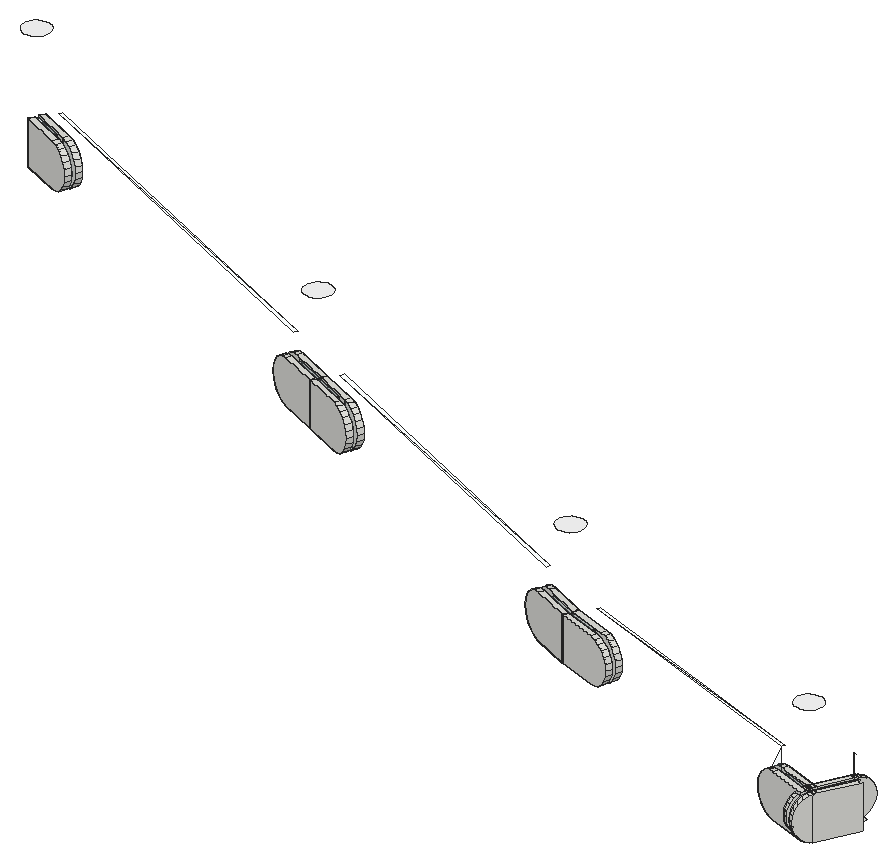
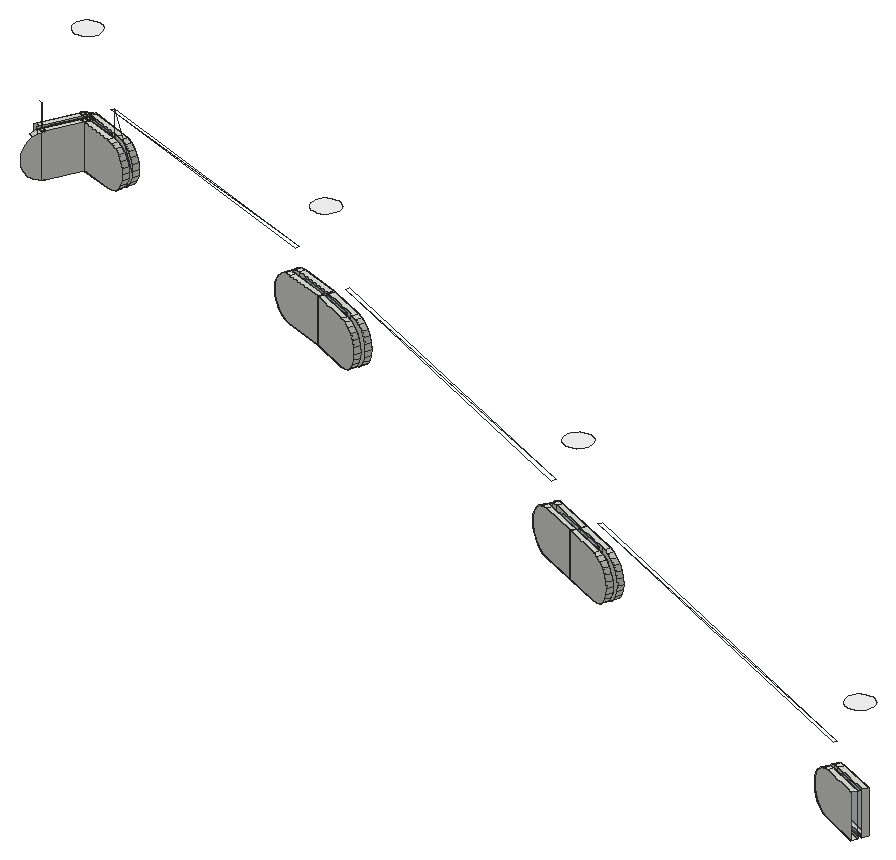
# SketchUp Ruby script. Lengths in inches.
U = 1.inch
M = Sketchup.active_model
def pt(a) = Geom::Point3d.new(a.map { |v| v * U })
def face(e, loops, mat)
  f = e.add_face(loops[0].map { |a| pt(a) })
  loops[1..].each { |l| e.add_face(l.map { |a| pt(a) }).erase! }
  f.material = f.back_material = mat if mat
  f
end
# faces: each face lists its corners as indices into pts; further lists are holes
def faces(e, pts, list, mat = nil) = list.each { |f| face(e, (f[0].is_a?(Array) ? f : [f]).map { |l| l.map { |i| pts[i] } }, mat) }
# xy, xz, yz: faces in a plane at the given z, y or x. An outline is a flat list of corners, or four numbers for a rectangle; further outlines are holes
def ring(l) = l.size == 4 ? [[l[0], l[1]], [l[2], l[1]], [l[2], l[3]], [l[0], l[3]]] : l.each_slice(2).to_a
def flat(e, list, mat, &to3) = list.each { |f| face(e, (f[0].is_a?(Array) ? f : [f]).map { |l| ring(l).map { |u, v| to3.(u, v) } }, mat) }
def xy(e, z, list, mat = nil) = flat(e, list, mat) { |x, y| [x, y, z] }
def xz(e, y, list, mat = nil) = flat(e, list, mat) { |x, z| [x, y, z] }
def yz(e, x, list, mat = nil) = flat(e, list, mat) { |y, z| [x, y, z] }
def lines(e, pts, list) = list.each { |a, b| e.add_line(pt(pts[a]), pt(pts[b])) }
# prism: a flat outline (further loops are holes) pulled along v
def prism(e, loops, v, mat = nil)
  f = face(e, loops, mat); d = Geom::Vector3d.new(v.map { |x| x * U })
  f.pushpull(f.normal.samedirection?(d) ? d.length : -d.length)
end
def box(e, o, s, mat = nil) = prism(e, [[o, [o[0] + s[0], o[1], o[2]], [o[0] + s[0], o[1] + s[1], o[2]], [o[0], o[1] + s[1], o[2]]]], [0, 0, s[2]], mat)
def at(x, y, z, deg = 0) = Geom::Transformation.translation(pt([x, y, z])) * Geom::Transformation.rotation(ORIGIN, Z_AXIS, deg.degrees)
def axes(o, x, y, z) = Geom::Transformation.new([*x, 0, *y, 0, *z, 0, *pt(o).to_a, 1])
def part(name) = M.definitions.add(name)
# library, detail: a bought-in or finely detailed component or shape, given as its bounding box
def library(name, o, s) = part(name).tap { |d| box(d.entities, o, s) }
def detail(e, o, s) = box(e.add_group.entities, o, s)
def put(e, d, t, mat = nil) = e.add_instance(d, t).tap { |i| i.material = mat if mat }
def group(e, t, mat = nil) = e.add_group.tap { |g| g.transformation = t; g.material = mat if mat }.entities
root = M.entities
M.materials.add("Glass_Safety_01").color = [204, 235, 244]
M.materials["Glass_Safety_01"].alpha = 0.1
M.materials.add("[Color_000]").color = [255, 255, 255]
xy(root,351.283,[[842.969,535.471,841.097,536.081,841.182,536.343,841.404,536.271,843.054,535.733],[843.42,535.662,843.173,535.784,843.242,535.924,843.489,535.803],[843.489,535.803,843.242,535.924,844.039,537.551,844.286,537.43],[842.996,535.87,842.749,535.992,842.769,536.033,843.034,535.947,843.115,535.921,843.2,536.183,843.156,536.197,842.891,536.283,843.615,537.759,843.862,537.638,843.156,536.197,843.065,536.011,843.034,535.947],[843.115,535.921,843.034,535.947,843.065,536.011,843.156,536.197,843.2,536.183],
  [843.034,535.947,842.769,536.033,842.817,536.132,843.065,536.011],[843.065,536.011,842.817,536.132,842.891,536.283,843.156,536.197],[842.769,536.033,841.465,536.458,841.243,536.53,841.329,536.792,842.891,536.283,842.817,536.132],[843.862,537.638,843.615,537.759,843.677,537.885,843.929,537.775,843.867,537.648],[843.929,537.775,843.677,537.885,843.68,537.892,843.684,537.9,843.931,537.779],
  [829.024,540.014,827.152,540.623,827.238,540.885,829.109,540.276],[829.17,540.463,827.307,541.069,827.417,541.322,827.401,541.329,829.256,540.725],[827.119,540.636,825.314,541.422,825.424,541.675,825.595,541.6,827.229,540.889],[827.307,541.069,827.299,541.073,827.384,541.335,827.401,541.329,827.417,541.322],[827.299,541.073,825.674,541.78,825.503,541.855,825.613,542.108,827.401,541.329,827.384,541.335],
  [809.928,548.122,808.124,548.907,808.234,549.16,810.038,548.374],[810.117,548.555,808.312,549.341,808.422,549.593,810.227,548.807],[808.124,548.907,806.319,549.693,806.429,549.946,806.582,549.879,808.234,549.16],[808.312,549.341,806.661,550.06,806.507,550.127,806.617,550.379,808.422,549.593],[788.708,557.364,786.903,558.15,787.013,558.402,788.818,557.616],
  [788.896,557.797,787.092,558.583,787.202,558.835,789.006,558.049]])
xy(root,351.362,[[843.054,535.733,841.557,536.221,841.618,536.408,843.034,535.947,842.996,535.87,843.084,535.827],[843.173,535.784,843.084,535.827,843.115,535.921,843.034,535.947,843.238,536.364,843.415,536.278],[843.084,535.827,842.996,535.87,843.034,535.947,843.115,535.921],[843.415,536.278,843.238,536.364,843.689,537.285,843.866,537.198],[828.735,540.398,827.238,540.885,827.268,540.979,827.307,541.069,828.796,540.585],
  [827.229,540.889,825.785,541.517,825.864,541.698,827.299,541.073,827.268,540.979],[827.268,540.979,827.299,541.073,827.307,541.069],[809.677,548.531,808.234,549.16,808.312,549.341,809.756,548.712],[808.234,549.16,806.79,549.789,806.868,549.969,808.312,549.341],[788.457,557.773,787.013,558.402,787.092,558.583,788.535,557.954]],"Glass_Safety_01")
xy(root,353.33,[[843.054,535.733,843.084,535.827,842.996,535.87,843.034,535.947,841.618,536.408,841.557,536.221],[843.173,535.784,843.415,536.278,843.238,536.364,843.034,535.947,843.115,535.921,843.084,535.827],[843.084,535.827,843.115,535.921,843.034,535.947,842.996,535.87],[843.415,536.278,843.866,537.198,843.689,537.285,843.238,536.364],[843.866,537.198,844.039,537.551,844.044,537.561,844.108,537.692,844.019,537.735,843.929,537.775,843.867,537.648,843.862,537.638,843.689,537.285],
  [828.735,540.398,828.796,540.585,827.307,541.069,827.268,540.979,827.238,540.885],[827.229,540.889,827.268,540.979,827.299,541.073,825.864,541.698,825.785,541.517],[827.268,540.979,827.307,541.069,827.299,541.073],[809.677,548.531,809.756,548.712,808.312,549.341,808.234,549.16],[808.234,549.16,808.312,549.341,806.868,549.969,806.79,549.789],
  [788.457,557.773,788.535,557.954,787.092,558.583,787.013,558.402]],"Glass_Safety_01")
xy(root,353.409,[[842.969,535.471,843.054,535.733,841.404,536.271,841.182,536.343,841.097,536.081],[843.42,535.662,843.489,535.803,843.242,535.924,843.173,535.784],[843.489,535.803,844.286,537.43,844.039,537.551,843.242,535.924],[842.996,535.87,843.034,535.947,843.065,536.011,843.156,536.197,843.862,537.638,843.615,537.759,842.891,536.283,843.156,536.197,843.2,536.183,843.115,535.921,843.034,535.947,842.769,536.033,842.749,535.992],[843.115,535.921,843.2,536.183,843.156,536.197,843.065,536.011,843.034,535.947],
  [843.034,535.947,843.065,536.011,842.817,536.132,842.769,536.033],[843.065,536.011,843.156,536.197,842.891,536.283,842.817,536.132],[842.769,536.033,842.817,536.132,842.891,536.283,841.329,536.792,841.243,536.53,841.465,536.458],[843.862,537.638,843.867,537.648,843.929,537.775,843.677,537.885,843.615,537.759],[843.929,537.775,843.931,537.779,843.684,537.9,843.68,537.892,843.677,537.885],
  [829.024,540.014,829.109,540.276,827.238,540.885,827.152,540.623],[829.17,540.463,829.256,540.725,827.401,541.329,827.417,541.322,827.307,541.069],[827.119,540.636,827.229,540.889,825.595,541.6,825.424,541.675,825.314,541.422],[827.307,541.069,827.417,541.322,827.401,541.329,827.384,541.335,827.299,541.073],[827.299,541.073,827.384,541.335,827.401,541.329,825.613,542.108,825.503,541.855,825.674,541.78],
  [809.928,548.122,810.038,548.374,808.234,549.16,808.124,548.907],[810.117,548.555,810.227,548.807,808.422,549.593,808.312,549.341],[808.124,548.907,808.234,549.16,806.582,549.879,806.429,549.946,806.319,549.693],[808.312,549.341,808.422,549.593,806.617,550.379,806.507,550.127,806.661,550.06],[788.708,557.364,788.818,557.616,787.013,558.402,786.903,558.15],
  [788.896,557.797,789.006,558.049,787.202,558.835,787.092,558.583]])
xy(root,354.511,[[841.404,536.271,841.465,536.458,829.109,540.276],[841.465,536.458,829.17,540.463,829.109,540.276],[844.039,537.551,843.867,537.648,843.862,537.638],[825.595,541.6,825.674,541.78,810.038,548.374],[825.674,541.78,810.117,548.555,810.038,548.374],
  [806.582,549.879,806.661,550.06,788.818,557.616],[806.661,550.06,788.896,557.797,788.818,557.616]],"Glass_Safety_01")
xy(root,357.267,[[843.13,535.199,843.291,535.232,843.4375,535.305,843.561,535.415,843.651,535.552,843.703,535.708,843.713,535.872,843.68,536.033,843.606,536.18,843.497,536.303,843.36,536.394,843.204,536.446,843.039,536.455,842.878,536.422,842.731,536.349,842.608,536.239,842.518,536.102,842.466,535.946,842.456,535.782,842.489,535.621,842.563,535.474,842.672,535.351,842.809,535.26,842.965,535.208],[827.313,540.351,827.474,540.384,827.621,540.457,827.744,540.567,827.835,540.704,827.887,540.86,827.896,541.024,827.863,541.185,827.79,541.332,827.681,541.455,827.543,541.546,827.387,541.598,827.223,541.607,827.062,541.574,826.915,541.501,826.792,541.391,826.701,541.254,826.65,541.098,826.64,540.934,826.673,540.773,826.747,540.626,826.856,540.503,826.993,540.412,827.149,540.36],[808.318,548.622,808.479,548.655,808.626,548.729,808.749,548.838,808.84,548.975,808.891,549.131,808.901,549.295,808.868,549.456,808.794,549.603,808.685,549.726,808.548,549.817,808.392,549.869,808.228,549.879,808.067,549.846,807.92,549.772,807.797,549.663,807.706,549.525,807.654,549.369,807.645,549.205,807.678,549.044,807.751,548.897,807.86,548.774,807.998,548.684,808.154,548.632],[787.097,557.864,787.258,557.897,787.405,557.971,787.528,558.08,787.619,558.217,787.671,558.373,787.681,558.538,787.648,558.699,787.574,558.846,787.465,558.969,787.327,559.059,787.171,559.111,787.007,559.121,786.846,559.088,786.699,559.014,786.576,558.905,786.486,558.768,786.434,558.612,786.424,558.447,786.457,558.286,786.531,558.139,786.64,558.016,786.777,557.926,786.933,557.874]],"[Color_000]")
p = [[843.368,535.556,351.319],[843.42,535.662,351.304],[843.42,535.662,353.388],[843.368,535.556,353.373],[843.255,535.326,353.267],[843.158,535.128,353.098],
  [843.084,534.976,352.877],[843.037,534.881,352.621],[843.021,534.848,352.346],[843.037,534.881,352.071],[843.084,534.976,351.815],[843.158,535.128,351.594],
  [843.255,535.326,351.425],[843.121,535.677,353.373],[843.173,535.784,353.388],[843.173,535.784,353.33],[843.173,535.784,351.362],[843.173,535.784,351.304],
  [843.121,535.677,351.319],[843.008,535.447,351.425],[842.911,535.249,351.594],[842.837,535.098,351.815],[842.79,535.002,352.071],[842.774,534.97,352.346],
  [842.79,535.002,352.621],[842.837,535.098,352.877],[842.911,535.249,353.098],[843.008,535.447,353.267],[843.862,537.638,351.283],[843.863,537.64,351.283],
  [843.867,537.648,351.283],[843.929,537.775,351.283],[843.929,537.775,351.303],[843.929,537.775,351.362],[843.929,537.775,353.33],[843.929,537.775,353.389],
  [843.929,537.775,353.409],[843.867,537.648,353.409],[843.862,537.638,353.409],[843.156,536.197,353.409],[843.065,536.011,353.409],[842.996,535.87,353.388],
  [842.944,535.764,353.373],[842.831,535.534,353.267],[842.734,535.336,353.098],[842.66,535.184,352.877],[842.613,535.089,352.621],[842.597,535.056,352.346],
  [842.613,535.089,352.071],[842.66,535.184,351.815],[842.734,535.336,351.594],[842.831,535.534,351.425],[842.944,535.764,351.319],[842.996,535.87,351.304],
  [843.065,536.011,351.283],[843.156,536.197,351.283],[842.696,535.885,353.373],[842.749,535.992,353.388],[842.749,535.992,351.304],[842.696,535.885,351.319],
  [842.584,535.655,351.425],[842.487,535.457,351.594],[842.412,535.305,351.815],[842.366,535.21,352.071],[842.35,535.178,352.346],[842.366,535.21,352.621],
  [842.412,535.305,352.877],[842.487,535.457,353.098],[842.584,535.655,353.267],[842.969,535.471,353.409],[841.097,536.081,353.409],[840.835,536.166,353.373],
  [840.592,536.246,353.267],[840.382,536.314,353.098],[840.222,536.366,352.877],[840.121,536.399,352.621],[840.086,536.41,352.346],[840.121,536.399,352.071],
  [840.222,536.366,351.815],[840.382,536.314,351.594],[840.592,536.246,351.425],[840.835,536.166,351.319],[841.097,536.081,351.283],[842.969,535.471,351.283],
  [843.054,535.733,351.283],[843.054,535.733,351.362],[843.054,535.733,353.33],[843.054,535.733,353.409],[843.242,535.924,351.283],[843.489,535.803,351.283],
  [841.404,536.271,351.283],[841.404,536.271,353.409],[841.557,536.221,353.33],[841.557,536.221,351.362],[843.173,535.784,351.283],[843.42,535.662,351.283],
  [843.42,535.662,353.409],[843.173,535.784,353.409],[844.286,537.43,351.283],[844.355,537.571,351.304],[844.355,537.571,353.388],[844.286,537.43,353.409],
  [843.489,535.803,353.409],[842.817,536.132,351.283],[843.415,536.278,351.362],[843.415,536.278,353.33],[843.242,535.924,353.409],[844.039,537.551,353.409],
  [844.044,537.561,353.409],[844.044,537.561,353.408],[844.039,537.551,353.33],[844.044,537.561,353.33],[844.108,537.692,353.388],[844.108,537.692,353.33],
  [844.044,537.562,351.362],[844.108,537.692,351.362],[844.108,537.692,351.304],[844.044,537.562,351.285],[844.044,537.562,351.283],[844.043,537.56,351.283],
  [844.043,537.56,351.284],[844.043,537.56,351.362],[844.039,537.551,351.362],[844.039,537.551,351.283],[843.866,537.198,351.362],[843.866,537.198,353.33],
  [842.769,536.033,353.409],[841.465,536.458,353.409],[841.465,536.458,351.283],[842.769,536.033,351.283],[843.034,535.947,351.283],[843.115,535.921,351.283],
  [843.115,535.921,351.362],[843.034,535.947,351.362],[841.618,536.408,351.362],[841.618,536.408,353.33],[843.034,535.947,353.33],[843.115,535.921,353.33],
  [843.115,535.921,353.409],[843.034,535.947,353.409],[842.996,535.87,351.283],[842.996,535.87,351.362],[842.996,535.87,353.33],[842.996,535.87,353.409],
  [842.749,535.992,353.409],[842.749,535.992,351.283],[843.862,537.638,351.362],[843.689,537.285,351.362],[843.238,536.364,351.362],[843.2,536.183,351.283],
  [843.2,536.183,353.409],[843.615,537.759,353.409],[843.676,537.885,353.391],[843.676,537.885,351.301],[843.615,537.759,351.283],[842.891,536.283,351.283],
  [842.817,536.132,353.409],[842.891,536.283,353.409],[840.921,536.428,351.319],[841.182,536.343,351.283],[841.329,536.792,351.283],[841.067,536.878,351.319],
  [840.823,536.957,351.425],[840.614,537.025,351.594],[840.453,537.077,351.815],[840.352,537.11,352.071],[840.318,537.122,352.346],[840.352,537.11,352.621],
  [840.453,537.077,352.877],[840.614,537.025,353.098],[840.823,536.957,353.267],[841.067,536.878,353.373],[841.329,536.792,353.409],[840.677,536.508,351.425],
  [840.468,536.576,351.594],[840.307,536.628,351.815],[840.206,536.661,352.071],[840.182,536.669,352.264],[840.743,536.486,353.295],[840.921,536.428,353.373],
  [841.182,536.343,353.409],[841.243,536.53,351.283],[841.243,536.53,353.409],[840.982,536.616,353.373],[840.738,536.695,353.267],[840.529,536.763,353.098],
  [840.368,536.815,352.877],[840.267,536.848,352.621],[840.233,536.86,352.346],[840.267,536.848,352.071],[840.368,536.815,351.815],[840.529,536.763,351.594],
  [840.738,536.695,351.425],[840.982,536.616,351.319],[843.983,537.885,351.319],[843.931,537.779,351.304],[843.867,537.648,351.285],[843.684,537.9,351.304],
  [843.736,538.006,351.319],[843.863,537.64,351.362],[843.867,537.648,351.362],[843.677,537.885,351.283],[843.677,537.885,353.409],[843.931,537.779,351.283],
  [843.684,537.9,351.283],[843.684,537.9,353.388],[843.684,537.9,353.409],[843.931,537.779,353.409],[843.931,537.779,353.388],[843.931,537.779,353.33],
  [843.931,537.779,351.362],[843.68,537.892,351.283],[844.096,538.115,351.425],[843.849,538.237,351.425],[843.736,538.006,353.373],[843.849,538.237,353.267],
  [843.945,538.434,353.098],[844.02,538.586,352.877],[844.066,538.681,352.621],[844.082,538.714,352.346],[844.066,538.681,352.071],[844.02,538.586,351.815],
  [843.945,538.434,351.594],[829.024,540.014,353.409],[827.152,540.623,353.409],[827.152,540.623,351.283],[829.024,540.014,351.283],[829.286,539.928,351.319],
  [829.529,539.849,351.425],[829.739,539.781,351.594],[829.899,539.729,351.815],[830,539.696,352.071],[830.035,539.684,352.346],[830,539.696,352.621],
  [829.899,539.729,352.877],[829.739,539.781,353.098],[829.529,539.849,353.267],[829.286,539.928,353.373],[829.371,540.19,351.319],[829.615,540.111,351.425],
  [829.109,540.276,351.283],[829.109,540.276,353.409],[829.824,540.043,351.594],[829.985,539.991,351.815],[830.086,539.958,352.071],[830.12,539.946,352.346],
  [830.086,539.958,352.621],[829.985,539.991,352.877],[829.824,540.043,353.098],[829.615,540.111,353.267],[829.371,540.19,353.373],[827.307,541.069,353.409],
  [827.299,541.073,353.409],[827.299,541.073,353.33],[827.299,541.073,351.362],[827.299,541.073,351.283],[827.307,541.069,351.283],[829.17,540.463,351.283],
  [829.432,540.378,351.319],[829.676,540.298,351.425],[829.885,540.23,351.594],[830.046,540.178,351.815],[830.147,540.145,352.071],[830.181,540.134,352.346],
  [830.147,540.145,352.621],[830.046,540.178,352.877],[829.885,540.23,353.098],[829.676,540.298,353.267],[829.432,540.378,353.373],[829.17,540.463,353.409],
  [827.238,540.885,353.409],[827.238,540.885,351.283],[827.238,540.885,351.362],[828.735,540.398,351.362],[828.735,540.398,353.33],[827.238,540.885,353.33],
  [829.517,540.64,351.319],[829.761,540.56,351.425],[827.384,541.335,353.409],[827.401,541.329,353.409],[829.256,540.725,353.409],[829.517,540.64,353.373],
  [829.761,540.56,353.267],[829.97,540.492,353.098],[830.131,540.44,352.877],[830.232,540.407,352.621],[830.266,540.396,352.346],[830.232,540.407,352.071],
  [830.131,540.44,351.815],[829.97,540.492,351.594],[829.256,540.725,351.283],[827.401,541.329,351.283],[827.384,541.335,351.283],[827.119,540.636,353.409],
  [825.314,541.422,353.409],[825.062,541.532,353.373],[824.827,541.634,353.267],[824.625,541.722,353.098],[824.47,541.789,352.877],[824.373,541.832,352.621],
  [824.339,541.846,352.346],[824.373,541.832,352.071],[824.47,541.789,351.815],[824.625,541.722,351.594],[824.827,541.634,351.425],[825.062,541.532,351.319],
  [825.314,541.422,351.283],[827.119,540.636,351.283],[827.229,540.889,351.283],[827.229,540.889,351.362],[827.229,540.889,353.33],[827.229,540.889,353.409],
  [825.595,541.6,351.283],[825.595,541.6,353.409],[825.785,541.517,353.33],[825.785,541.517,351.362],[825.503,541.855,351.283],[825.674,541.78,351.283],
  [825.674,541.78,353.409],[825.503,541.855,353.409],[825.25,541.965,353.373],[825.015,542.067,353.267],[824.813,542.155,353.098],[824.659,542.223,352.877],
  [824.561,542.265,352.621],[824.528,542.279,352.346],[824.561,542.265,352.071],[824.659,542.223,351.815],[824.813,542.155,351.594],[825.015,542.067,351.425],
  [825.25,541.965,351.319],[827.307,541.069,351.362],[827.307,541.069,353.33],[827.417,541.322,351.283],[827.417,541.322,353.409],[825.613,542.108,351.283],
  [825.36,542.218,351.319],[825.125,542.32,351.425],[824.923,542.408,351.594],[824.769,542.475,351.815],[824.671,542.518,352.071],[824.638,542.532,352.346],
  [824.671,542.518,352.621],[824.769,542.475,352.877],[824.923,542.408,353.098],[825.125,542.32,353.267],[825.36,542.218,353.373],[825.613,542.108,353.409],
  [825.172,541.784,351.319],[825.424,541.675,351.283],[824.937,541.887,351.425],[825.424,541.675,353.409],[824.735,541.975,351.594],[824.58,542.042,351.815],
  [824.483,542.085,352.071],[824.449,542.099,352.346],[824.483,542.085,352.621],[824.58,542.042,352.877],[824.735,541.975,353.098],[824.937,541.887,353.267],
  [825.172,541.784,353.373],[809.928,548.122,353.409],[808.124,548.907,353.409],[808.124,548.907,351.283],[809.928,548.122,351.283],[810.181,548.012,351.319],
  [810.416,547.909,351.425],[810.618,547.821,351.594],[810.772,547.754,351.815],[810.87,547.712,352.071],[810.903,547.697,352.346],[810.87,547.712,352.621],
  [810.772,547.754,352.877],[810.618,547.821,353.098],[810.416,547.909,353.267],[810.181,548.012,353.373],[810.038,548.374,353.409],[810.038,548.374,351.283],
  [810.291,548.264,351.319],[810.526,548.162,351.425],[810.728,548.074,351.594],[810.882,548.007,351.815],[810.98,547.964,352.071],[811.013,547.95,352.346],
  [810.98,547.964,352.621],[810.882,548.007,352.877],[810.728,548.074,353.098],[810.526,548.162,353.267],[810.291,548.264,353.373],[810.117,548.555,351.283],
  [810.117,548.555,353.409],[810.369,548.445,353.373],[810.604,548.342,353.267],[810.806,548.255,353.098],[810.961,548.187,352.877],[811.058,548.145,352.621],
  [811.092,548.13,352.346],[811.058,548.145,352.071],[810.961,548.187,351.815],[810.806,548.255,351.594],[810.604,548.342,351.425],[810.369,548.445,351.319],
  [810.479,548.698,351.319],[810.714,548.595,351.425],[808.234,549.16,353.409],[808.234,549.16,351.283],[808.234,549.16,351.362],[809.677,548.531,351.362],
  [809.677,548.531,353.33],[808.234,549.16,353.33],[808.422,549.593,353.409],[810.227,548.807,353.409],[810.479,548.698,353.373],[810.714,548.595,353.267],
  [810.916,548.507,353.098],[811.071,548.44,352.877],[811.168,548.397,352.621],[811.202,548.383,352.346],[811.168,548.397,352.071],[811.071,548.44,351.815],
  [810.916,548.507,351.594],[810.227,548.807,351.283],[808.422,549.593,351.283],[808.312,549.341,351.283],[808.312,549.341,353.409],[808.312,549.341,353.33],
  [809.756,548.712,353.33],[809.756,548.712,351.362],[808.312,549.341,351.362],[806.319,549.693,353.409],[806.067,549.803,353.373],[805.831,549.906,353.267],
  [805.63,549.994,353.098],[805.475,550.061,352.877],[805.377,550.103,352.621],[805.344,550.118,352.346],[805.377,550.103,352.071],[805.475,550.061,351.815],
  [805.63,549.994,351.594],[805.831,549.906,351.425],[806.067,549.803,351.319],[806.319,549.693,351.283],[806.582,549.879,351.283],[806.582,549.879,353.409],
  [806.79,549.789,353.33],[806.79,549.789,351.362],[806.661,550.06,353.409],[806.661,550.06,351.283],[806.868,549.969,351.362],[806.868,549.969,353.33],
  [806.617,550.379,353.409],[806.617,550.379,351.283],[806.365,550.489,351.319],[806.13,550.591,351.425],[805.928,550.679,351.594],[805.773,550.747,351.815],
  [805.676,550.789,352.071],[805.643,550.804,352.346],[805.676,550.789,352.621],[805.773,550.747,352.877],[805.928,550.679,353.098],[806.13,550.591,353.267],
  [806.365,550.489,353.373],[806.177,550.056,351.319],[806.429,549.946,351.283],[805.942,550.158,351.425],[806.429,549.946,353.409],[805.74,550.246,351.594],
  [805.585,550.314,351.815],[805.487,550.356,352.071],[805.454,550.371,352.346],[805.487,550.356,352.621],[805.585,550.314,352.877],[805.74,550.246,353.098],
  [805.942,550.158,353.267],[806.177,550.056,353.373],[806.507,550.127,351.283],[806.507,550.127,353.409],[806.255,550.236,353.373],[806.02,550.339,353.267],
  [805.818,550.427,353.098],[805.663,550.494,352.877],[805.566,550.537,352.621],[805.533,550.551,352.346],[805.566,550.537,352.071],[805.663,550.494,351.815],
  [805.818,550.427,351.594],[806.02,550.339,351.425],[806.255,550.236,351.319],[788.708,557.364,353.409],[786.903,558.15,353.409],[786.903,558.15,351.283],
  [788.708,557.364,351.283],[788.96,557.254,351.319],[789.195,557.151,351.425],[789.397,557.063,351.594],[789.552,556.996,351.815],[789.649,556.954,352.071],
  [789.682,556.939,352.346],[789.649,556.954,352.621],[789.552,556.996,352.877],[789.397,557.063,353.098],[789.195,557.151,353.267],[788.96,557.254,353.373],
  [788.818,557.616,353.409],[788.818,557.616,351.283],[789.07,557.506,351.319],[789.305,557.404,351.425],[789.507,557.316,351.594],[789.662,557.249,351.815],
  [789.759,557.206,352.071],[789.792,557.192,352.346],[789.759,557.206,352.621],[789.662,557.249,352.877],[789.507,557.316,353.098],[789.305,557.404,353.267],
  [789.07,557.506,353.373],[788.896,557.797,351.283],[788.896,557.797,353.409],[789.149,557.687,353.373],[789.384,557.585,353.267],[789.586,557.497,353.098],
  [789.74,557.429,352.877],[789.838,557.387,352.621],[789.871,557.372,352.346],[789.838,557.387,352.071],[789.74,557.429,351.815],[789.586,557.497,351.594],
  [789.384,557.585,351.425],[789.149,557.687,351.319],[787.013,558.402,353.409],[787.013,558.402,351.283],[787.013,558.402,351.362],[788.457,557.773,351.362],
  [788.457,557.773,353.33],[787.013,558.402,353.33],[787.202,558.835,353.409],[789.006,558.049,353.409],[789.259,557.94,353.373],[789.494,557.837,353.267],
  [789.696,557.749,353.098],[789.85,557.682,352.877],[789.948,557.639,352.621],[789.981,557.625,352.346],[789.948,557.639,352.071],[789.85,557.682,351.815],
  [789.696,557.749,351.594],[789.494,557.837,351.425],[789.259,557.94,351.319],[789.006,558.049,351.283],[787.202,558.835,351.283],[787.092,558.583,351.283],
  [787.092,558.583,353.409],[787.092,558.583,353.33],[788.535,557.954,353.33],[788.535,557.954,351.362],[787.092,558.583,351.362],[843.084,535.827,351.362],
  [843.084,535.827,353.33],[843.238,536.364,353.33],[843.689,537.285,353.33],[843.862,537.638,353.33],[843.867,537.648,353.33],[843.93,537.777,353.33],
  [843.93,537.777,351.362],[828.796,540.585,351.362],[828.796,540.585,353.33],[827.268,540.979,353.33],[827.268,540.979,351.362],[825.864,541.698,353.33],
  [825.864,541.698,351.362],[827.303,541.071,353.33],[827.303,541.071,351.362],[840.172,536.672,352.346],[840.206,536.661,352.621],[840.307,536.628,352.877],
  [840.468,536.576,353.098],[840.677,536.508,353.267],[841.404,536.271,354.511],[843.867,537.648,353.407],[843.983,537.885,353.373],[844.096,538.115,353.267],
  [843.862,537.638,354.511],[843.867,537.648,354.511],[843.68,537.892,353.409]]
faces(root,p,[[0,1,2,3,4,5,6,7,8,9,10,11,12],[13,14,15,16,17,18,19,20,21,22,23,24,25,26,27],[28,29,30,31,32,33,34,35,36,37,38,39,40,41,42,43,44,45,46,47,48,49,50,51,52,53,54,55],[56,57,58,59,60,61,62,63,64,65,66,67,68],[19,18,0,12],[69,70,71,72,73,74,75,76,77,78,79,80,81,82,83],[52,51,60,59],[84,85,86,87,69,83],
  [18,17,88,89,1,0],[84,90,91,87,86,92,93,85],[17,94,95,1,2,96,97,14,15,16],[95,89,1],[2,1,89,98,99,100,101,102],[53,52,59,58,103,54],[94,17,88],[[88,17,16,104,105,15,14,106,107,108,109,107,110,111,109,112,113,111,114,115,116,117,118,119,120,121,122,123],[124,122,110,125]],
  [126,127,128,129,130,131,132,133,134,135,136,137,138,139],[140,53,141,142,41,143,144,57,58,145],[130,54,53,140],[55,28,146,147,148,133,141,53,54],[132,131,149,150,138,137],[145,58,103,129],[151,152,153,154,155,103,58,57,156,157],[158,159,82,81],
  [39,150,149,55,155,160,161,162,163,164,165,166,167,168,169,170,171,172,157],[173,158,81,80],[181,128,127,182,183,184,185,186,187,188,189,190,191,192,193],[181,193,161,160],[193,192,162,161],[194,195,32,196,29,28,154,153,197,198],[154,153,201],[31,32,33,34,35,36,202,152,153,201],
  [195,203,204,197,205,206,207,208,209,210],[209,208,35,34,33,32,195,210],[203,195,32,31],[211,201,153,197,204],[197,153,152,205],[212,194,198,213],[198,197,205,214,215,216,217,218,219,220,221,222,213],[223,224,225,226,227,228,229,230,231,232,233,234,235,236,237],
  [238,239,228,227],[240,238,227,226],[251,252,253,254,255,256,257,258,259,260,261,262,263,264,265,266,267,268,269],[270,241,240,271,272,273,274,275],[259,258,276,277],[278,279,280,281,282,283,284,285,286,287,288,289,277,276,290,291,292],[258,257,290,276],[293,294,295,296,297,298,299,300,301,302,303,304,305,306,307],
  [308,309,310,311,293,307],[272,271,225,224,270,275],[308,312,313,311,310,314,315,309],[316,317,255,254,253,252,318,319,320,321,322,323,324,325,326,327,328,329,330],[251,252,253,254,255,256,331,332],[331,256,333,334,251,332],[255,254,253,252,278,292],[279,334,333,291,335,336,337,338,339,340,341,342,343,344,345,346,347],
  [348,349,306,305],[350,348,305,304],[351,313,312,349,348,350,352,353,354,355,356,357,358,359,360],[316,330,336,335],[330,329,337,336],[361,362,363,364,365,366,367,368,369,370,371,372,373,374,375],[378,379,366,365],[377,378,365,364],
  [400,401,402,403],[404,376,377,405,406,407,408,409],[410,411,412,413,414,415,416,417,418,419,420,403,402,421,422],[401,389,421,402],[423,389,390,424,425,426,427,428],[362,429,430,431,432,433,434,435,436,437,438,439,440,441,363],[405,406,409,404,362,363],[405,442,443,404,409,444,445,406],
  [424,446,447,423,428,448,449,425],[428,423,422,410,424,425],[450,410,422,451,452,453,454,455,456,457,458,459,460,461,462],[463,464,441,440],[465,463,440,439],[466,443,442,464,463,465,467,468,469,470,471,472,473,474,475],[476,447,446,477,478,479,480,481,482,483,484,485,486,487,488],[476,488,452,451],
  [488,487,453,452],[489,490,491,492,493,494,495,496,497,498,499,500,501,502,503],[506,507,494,493],[505,506,493,492],[530,504,505,531,532,533,534,535],[536,537,538,539,540,541,542,543,544,545,546,547,548,549,550],[528,529,548,547],[529,517,549,548],
  [551,517,518,552,553,554,555,556],[531,532,535,530,490,491],[20,19,12,11],[51,50,61,60],[174,173,80,79],[192,191,163,162],[239,242,229,228],[260,259,277,289],
  [352,350,304,303],[329,328,338,337],[379,380,367,366],[399,400,403,420],[467,465,439,438],[487,486,454,453],[507,508,495,494],[527,528,547,546],
  [21,20,11,10],[50,49,62,61],[175,174,79,78],[191,190,164,163],[242,243,230,229],[261,260,289,288],[353,352,303,302],[328,327,339,338],
  [380,381,368,367],[398,399,420,419],[468,467,438,437],[486,485,455,454],[508,509,496,495],[526,527,546,545],[22,21,10,9],[49,48,63,62],
  [176,175,78,77],[190,189,165,164],[243,244,231,230],[262,261,288,287],[354,353,302,301],[327,326,340,339],[381,382,369,368],[397,398,419,418],
  [469,468,437,436],[485,484,456,455],[509,510,497,496],[525,526,545,544],[23,22,9,8],[48,47,64,63],[573,177,176,77,76],[189,188,166,165],
  [244,245,232,231],[263,262,287,286],[355,354,301,300],[326,325,341,340],[382,383,370,369],[396,397,418,417],[470,469,436,435],[484,483,457,456],
  [510,511,498,497],[524,525,544,543],[24,23,8,7],[47,46,65,64],[574,573,76,75],[177,573,574,575,576,577,178],[188,187,167,166],[245,246,233,232],
  [264,263,286,285],[356,355,300,299],[325,324,342,341],[383,384,371,370],[395,396,417,416],[471,470,435,434],[483,482,458,457],[511,512,499,498],
  [523,524,543,542],[25,24,7,6],[46,45,66,65],[575,574,75,74],[187,186,168,167],[246,247,234,233],[265,264,285,284],[357,356,299,298],
  [324,323,343,342],[384,385,372,371],[394,395,416,415],[472,471,434,433],[482,481,459,458],[512,513,500,499],[522,523,542,541],[26,25,6,5],
  [45,44,67,66],[576,575,74,73],[186,185,169,168],[247,248,235,234],[266,265,284,283],[358,357,298,297],[323,322,344,343],[385,386,373,372],
  [393,394,415,414],[473,472,433,432],[481,480,460,459],[513,514,501,500],[521,522,541,540],[27,26,5,4],[44,43,68,67],[577,576,73,72],
  [185,184,170,169],[248,249,236,235],[267,266,283,282],[359,358,297,296],[322,321,345,344],[386,387,374,373],[392,393,414,413],[474,473,432,431],
  [480,479,461,460],[514,515,502,501],[520,521,540,539],[13,27,4,3],[43,42,56,68],[136,559,560,561,38,39,40,41,142],[179,178,577,72,71],[184,183,171,170],
  [580,581,215,214],[249,250,237,236],[268,267,282,281],[360,359,296,295],[321,320,346,345],[387,388,375,374],[391,392,413,412],[475,474,431,430],
  [479,478,462,461],[515,516,503,502],[519,520,539,538],[106,14,13,3,2,102],[96,2,102],[41,40,156,57,56,42],[97,106,14],[143,41,40,139],
  [126,156,57,144],[180,179,71,70],[183,182,172,171],[38,579,35,208,580,214,205,152,151],[151,202,152],[36,35,208,207],[205,152,202,584,206],[250,241,223,237],
  [269,268,281,280],[351,360,295,294],[320,319,347,346],[388,376,361,375],[390,391,412,411],[466,475,430,429],[478,477,450,462],[516,504,489,503],
  [518,519,538,537]])
faces(root,p,[[91,90,159,158,173,174,175,176,177,178,179,180],[196,30,29,199,200],[241,240,238,239,242,243,244,245,246,247,248,249,250],[257,269,268,267,266,265,264,263,262,261,260,259,258],[376,377,378,379,380,381,382,383,384,385,386,387,388],[389,390,391,392,393,394,395,396,397,398,399,400,401],[504,505,506,507,508,509,510,511,512,513,514,515,516],[517,518,519,520,521,522,523,524,525,526,527,528,529],
  [92,86,85,93],[85,557,558,86],[557,558,142,141],[558,557,16,15],[137,558,557,132],[104,16,15,105],[137,136,135,134,133,132],[559,136,142,141,133,148],
  [135,134,93,92],[559,148,104,105],[125,105,104,124],[559,560,147,148],[124,147,560,125],[560,561,146,147],[199,146,561],[562,200,199,561],
  [33,200,562,34],[563,209,210,564,33,34],[275,274,273,272],[273,565,566,274],[565,331,332,566],[314,310,309,315],[567,568,272,275],[309,568,567,310],
  [332,567,568,331],[568,567,253,254],[569,253,254,570],[571,332,331,572,254,253],[569,570,315,314],[409,408,407,406],[427,426,408,407],[426,425,428,427],
  [444,409,406,445],[406,428,425,409],[425,449,448,428],[449,448,445,444],[535,534,533,532],[534,533,555,554],[554,553,556,555],[578,178,179,180,91],
  [561,38,579,562],[37,579,38,582,583]],"Glass_Safety_01")
